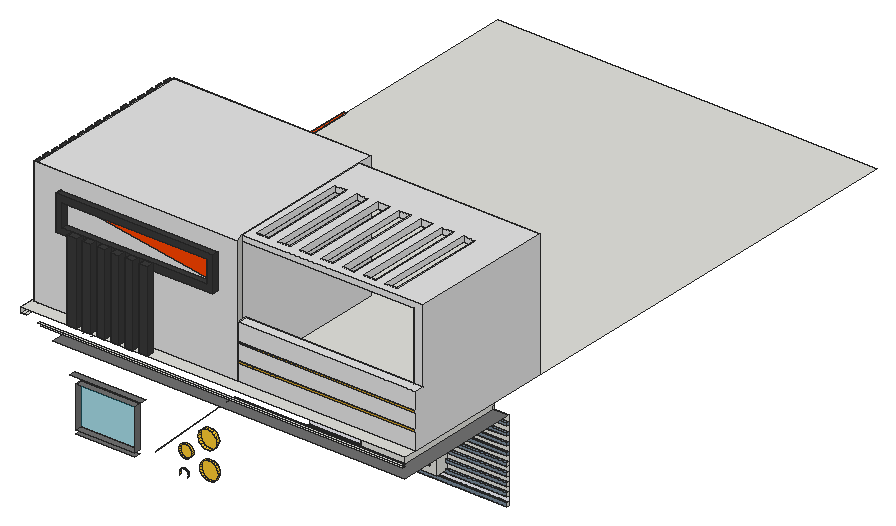
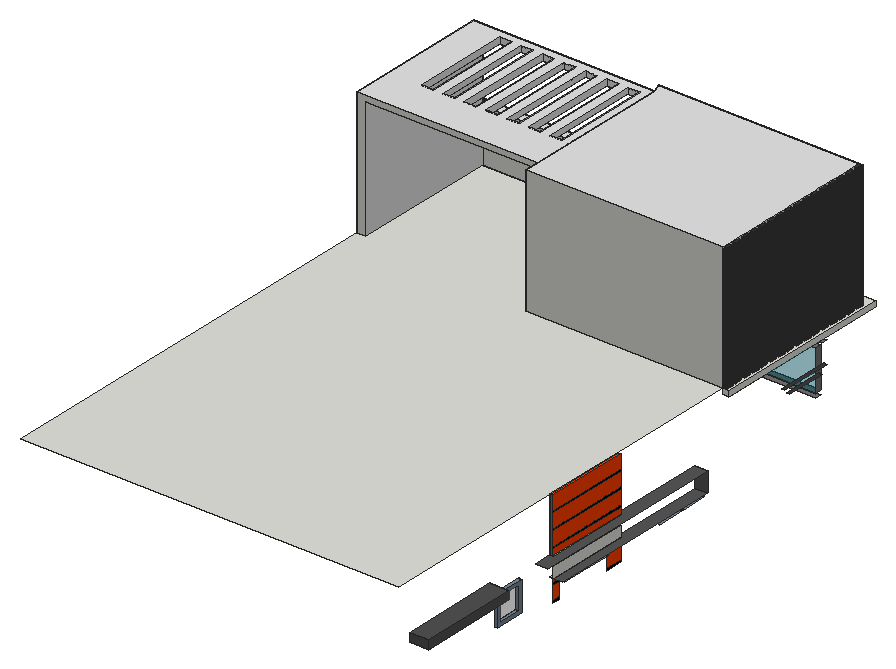
# SketchUp Ruby script. Lengths in inches.
U = 1.inch
M = Sketchup.active_model
def pt(a) = Geom::Point3d.new(a.map { |v| v * U })
def face(e, loops, mat)
  f = e.add_face(loops[0].map { |a| pt(a) })
  loops[1..].each { |l| e.add_face(l.map { |a| pt(a) }).erase! }
  f.material = f.back_material = mat if mat
  f
end
# faces: each face lists its corners as indices into pts; further lists are holes
def faces(e, pts, list, mat = nil) = list.each { |f| face(e, (f[0].is_a?(Array) ? f : [f]).map { |l| l.map { |i| pts[i] } }, mat) }
# xy, xz, yz: faces in a plane at the given z, y or x. An outline is a flat list of corners, or four numbers for a rectangle; further outlines are holes
def ring(l) = l.size == 4 ? [[l[0], l[1]], [l[2], l[1]], [l[2], l[3]], [l[0], l[3]]] : l.each_slice(2).to_a
def flat(e, list, mat, &to3) = list.each { |f| face(e, (f[0].is_a?(Array) ? f : [f]).map { |l| ring(l).map { |u, v| to3.(u, v) } }, mat) }
def xy(e, z, list, mat = nil) = flat(e, list, mat) { |x, y| [x, y, z] }
def xz(e, y, list, mat = nil) = flat(e, list, mat) { |x, z| [x, y, z] }
def yz(e, x, list, mat = nil) = flat(e, list, mat) { |y, z| [x, y, z] }
def lines(e, pts, list) = list.each { |a, b| e.add_line(pt(pts[a]), pt(pts[b])) }
# prism: a flat outline (further loops are holes) pulled along v
def prism(e, loops, v, mat = nil)
  f = face(e, loops, mat); d = Geom::Vector3d.new(v.map { |x| x * U })
  f.pushpull(f.normal.samedirection?(d) ? d.length : -d.length)
end
def box(e, o, s, mat = nil) = prism(e, [[o, [o[0] + s[0], o[1], o[2]], [o[0] + s[0], o[1] + s[1], o[2]], [o[0], o[1] + s[1], o[2]]]], [0, 0, s[2]], mat)
def at(x, y, z, deg = 0) = Geom::Transformation.translation(pt([x, y, z])) * Geom::Transformation.rotation(ORIGIN, Z_AXIS, deg.degrees)
def axes(o, x, y, z) = Geom::Transformation.new([*x, 0, *y, 0, *z, 0, *pt(o).to_a, 1])
def part(name) = M.definitions.add(name)
# library, detail: a bought-in or finely detailed component or shape, given as its bounding box
def library(name, o, s) = part(name).tap { |d| box(d.entities, o, s) }
def detail(e, o, s) = box(e.add_group.entities, o, s)
def put(e, d, t, mat = nil) = e.add_instance(d, t).tap { |i| i.material = mat if mat }
def group(e, t, mat = nil) = e.add_group.tap { |g| g.transformation = t; g.material = mat if mat }.entities
root = M.entities
M.materials.add("[0024_OrangeRed]").color = [255, 69, 0]
M.materials.add("[0045_Goldenrod]").color = [218, 165, 32]
M.materials.add("[0110_LightSlateGray]").color = [119, 136, 153]
M.materials.add("[0111_SlateGray]").color = [112, 128, 144]
M.materials.add("[0117_GhostWhite]").color = [248, 248, 255]
M.materials.add("[0135_DarkGray]").color = [81, 81, 81]
M.materials.add("[Color B05]").color = [255, 63, 0]
M.materials.add("[Color D04]").color = [255, 204, 50]
M.materials.add("[Color M05]").color = [114, 114, 114]
M.materials.add("[Color M06]").color = [86, 86, 86]
M.materials.add("[Color M07]").color = [58, 58, 58]
M.materials.add("[Color M09]").color = [0, 0, 0]
M.materials.add("[Polished Concrete Old]").color = [229, 229, 229]
M.materials.add("[Translucent Glass Gray]").color = [128, 128, 128]
M.materials["[Translucent Glass Gray]"].alpha = 0.5
M.materials.add("[Translucent Glass Tinted]").color = [4, 119, 142]
M.materials["[Translucent Glass Tinted]"].alpha = 0.48
xy(root,150.47,[[188.34,123.9375,363.6875,125.9375],[363.6875,123.9375,378,125.9375]],"[0110_LightSlateGray]")
xy(root,151.59,[[59.9,8,115.9,14]],"[Color M05]")
xy(root,153.53,[[188.34,123.9375,378,125.9375]],"[0110_LightSlateGray]")
xy(root,155.16,[[59.9,8,115.9,14]],"[Color M05]")
xy(root,159.03,[[188.34,123.9375,363.6875,125.9375],[363.6875,123.9375,378,125.9375]],"[0110_LightSlateGray]")
xy(root,160.2,[[246.52,113.9375,318.7,123.9375],[246.52,123.9375,318.7,125.9375]])
xy(root,161.99,[[15,420.33,18,448.89]],"[0110_LightSlateGray]")
xy(root,162.09,[[188.34,123.9375,246.52,125.9375],[318.7,123.9375,378,125.9375]],"[0110_LightSlateGray]")
xy(root,164.99,[[15,423.33,18,445.89]],"[0110_LightSlateGray]")
xy(root,165.42,[[15,203.12,18,226.79],[15,229.5,18,255.87]],"[0110_LightSlateGray]")
xy(root,166.2,[[252.52,113.9375,312.7,125.9375]])
xy(root,167.59,[[188.34,123.9375,246.52,125.9375],[318.7,123.9375,363.6875,125.9375],[363.6875,123.9375,378,125.9375]],"[0110_LightSlateGray]")
xy(root,168.375,[[12,321.75,15,345.13],[12,347.25,15,372.75]],"[0110_LightSlateGray]")
xy(root,168.42,[[15,200.12,18,258.87]],"[0110_LightSlateGray]")
xy(root,170.66,[[188.34,123.9375,246.52,125.9375],[318.7,123.9375,378,125.9375]],"[0110_LightSlateGray]")
xy(root,171.375,[[12,318.75,15,375.75]],"[0110_LightSlateGray]")
xy(root,174.92,[[15,302.36,18,382.63]])
xy(root,174.92,[[6,209.95,6,382.63,15,382.63,15,302.36,18,302.36,18,209.95]],"[Color M06]")
xy(root,176.15,[[188.34,123.9375,246.52,125.9375],[318.7,123.9375,363.6875,125.9375],[363.6875,123.9375,378,125.9375]],"[0110_LightSlateGray]")
xy(root,179.22,[[188.34,123.9375,246.52,125.9375]])
xy(root,179.22,[[318.7,123.9375,378,125.9375]],"[0110_LightSlateGray]")
xy(root,184.72,[[188.34,123.9375,246.52,125.9375],[318.7,123.9375,363.6875,125.9375],[363.6875,123.9375,378,125.9375]],"[0110_LightSlateGray]")
xy(root,187.55,[[15,423.33,18,445.89]])
xy(root,187.78,[[188.34,123.9375,246.52,125.9375]])
xy(root,187.78,[[318.7,123.9375,378,125.9375]],"[0110_LightSlateGray]")
xy(root,190.1,[[15,466.73,18,500.63],[15,503.73,18,540.73]],"[0135_DarkGray]")
xy(root,190.55,[[15,420.33,18,448.89]],"[0110_LightSlateGray]")
xy(root,193.1,[[0,453.79,0,549.98,18,549.98,18,543.73,15,543.73,15,463.73,18,463.73,18,453.79]],"[0135_DarkGray]")
xy(root,193.28,[[188.34,123.9375,246.52,125.9375],[318.7,123.9375,363.6875,125.9375],[363.6875,123.9375,378,125.9375]],"[0110_LightSlateGray]")
xy(root,194.12,[[59.9,8,115.9,14]],"[Color M05]")
xy(root,194.23,[[15,302.36,18,382.63]])
xy(root,194.23,[[6,209.95,18,209.95,18,302.36,15,302.36,15,382.63,18,382.63,18,399.82,6,399.82]],"[Color M06]")
xy(root,196.34,[[188.34,123.9375,246.52,125.9375]])
xy(root,196.34,[[318.7,123.9375,378,125.9375]],"[0110_LightSlateGray]")
xy(root,200.12,[[53.9,8,121.9,14]],"[Color M05]")
xy(root,201.17,[[0,453.79,18,549.98]],"[0135_DarkGray]")
xy(root,201.84,[[318.7,123.9375,363.6875,125.9375],[363.6875,123.9375,378,125.9375]],"[0110_LightSlateGray]")
xy(root,201.84,[[188.34,123.9375,246.52,125.9375]],"[0111_SlateGray]")
xy(root,203.27,[[252.52,113.9375,312.7,125.9375]])
xy(root,204.91,[[318.7,123.9375,378,125.9375]],"[0110_LightSlateGray]")
xy(root,204.91,[[188.34,123.9375,246.52,125.9375]],"[0111_SlateGray]")
xy(root,209.27,[[246.52,113.9375,318.7,125.9375]])
xy(root,210.4,[[188.34,123.9375,363.6875,125.9375],[363.6875,123.9375,378,125.9375]],"[0110_LightSlateGray]")
xy(root,211.37,[[12,66.99,15,104.86]],"[Color M07]")
xy(root,213.47,[[188.34,123.9375,378,125.9375]],"[0110_LightSlateGray]")
xy(root,217.37,[[12,60.99,15,110.86]],"[Color M07]")
xy(root,218.97,[[188.34,123.9375,363.6875,125.9375],[363.6875,123.9375,378,125.9375]],"[0110_LightSlateGray]")
xy(root,222.03,[[188.34,123.9375,378,125.9375]],"[0110_LightSlateGray]")
xy(root,227.53,[[188.34,123.9375,363.6875,125.9375]],"[0110_LightSlateGray]")
xy(root,227.53,[[42.91,2,42.91,14,201.375,14,201.375,20,363.6875,20,363.6875,125.9375,378,125.9375,378,2]],"[Color M05]")
xy(root,230.84,[[188.34,123.9375,363.6875,125.9375]])
xy(root,236.34,[[188.34,123.9375,363.6875,125.9375]],"[0110_LightSlateGray]")
xy(root,238.03,[[32.7,0,378,2]])
xy(root,239.39,[[30.46,0,378,2]])
xy(root,240,[[27,20,27,125.9375,188.34,125.9375,188.34,123.9375,363.6875,123.9375,363.6875,20]],"[Polished Concrete Old]")
xy(root,240.8125,[[12,2,15,175.3125],[15,2,18,175.3125],[12,175.3125,18,177.0625]])
xy(root,246,[[[12,2,378,2,378,14.84,15,14.84,15,21.19,18,21.19,18,25.15,15,25.15,15,31.5,18,31.5,18,35.46,15,35.46,15,41.81,18,41.81,18,45.78,15,45.78,15,52.13,18,52.13,18,56.09,15,56.09,15,62.44,18,62.44,18,66.4,15,66.4,15,72.75,18,72.75,18,76.71,15,76.71,15,83.06,18,83.06,18,87.03,15,87.03,15,93.38,18,93.38,18,97.34,15,97.34,15,103.69,18,103.69,18,107.65,15,107.65,15,114,18,114,18,117.96,15,117.96,15,124.31,18,124.31,18,128.28,15,128.28,15,134.63,18,134.63,18,138.59,15,138.59,15,144.94,18,144.94,18,148.9,15,148.9,15,155.25,18,155.25,18,159.21,15,159.21,15,165.56,18,165.56,18,169.53,15,169.53,15,175.88,18,175.88,18,176.98,205.83,176.98,205.83,23.84,209.18,23.84,209.18,24.34,369,24.34,369,162.88,378,162.88,378,563,18,563,18,177.0625,12,177.0625],[56.4375,2.09,66.15,8.84],[84.32,2.09,92.33,8.84],[97.82,2.09,105.83,8.84],[111.32,2.09,119.33,8.84],[124.82,2.09,132.83,8.84],[70.82,2.09,78.83,8.84]],[15,14.84,18,21.19],[18,14.84,27,23.84],[27,14.84,209.18,14.84,205.83,23.84,27,23.84],[209.18,14.84,209.18,23.84,205.83,23.84],
  [209.18,14.84,377.18,24.34],[377.18,14.84,378,24.34],[18,23.84,27,176.98],[27,23.84,205.83,176.98],[369,24.34,378,162.88],
  [15,25.15,18,31.5],[15,35.46,18,41.81],[15,45.78,18,52.13],[15,56.09,18,62.44],[15,66.4,18,72.75],
  [15,76.71,18,83.06],[15,87.03,18,93.38],[15,97.34,18,103.69],[15,107.65,18,114],[15,117.96,18,124.31],
  [15,128.28,18,134.63],[15,138.59,18,144.94],[15,148.9,18,155.25],[15,159.21,18,165.56],[15,169.53,18,175.88]])
xy(root,246,[[15,302.36,18,382.63]],"[0024_OrangeRed]")
xy(root,262.33,[[209.18,13.84,378,14.84]])
xy(root,264.09,[[209.18,13.84,378,14.84]])
xy(root,278.67,[[209.18,13.84,378,14.84]])
xy(root,280.32,[[209.18,13.84,378,14.84]])
xy(root,296.375,[[209.18,14.84,378,14.84,378,23.84,369.17,23.84,369,24.34,209.18,24.34]],"[Polished Concrete Old]")
xy(root,316.27,[[40.375,8.84,189.625,14.84]],"[Color M07]")
xy(root,322.27,[[56.4375,2.09,66.15,8.84],[70.82,2.09,78.83,8.84],[84.32,2.09,92.33,8.84],[97.82,2.09,105.83,8.84],[111.32,2.09,119.33,8.84],
  [124.82,2.09,132.83,8.84],[46.375,8.84,183.625,14.84]],"[Color M07]")
xy(root,343.64,[[46.375,8.84,183.625,14.84]],"[Color M07]")
xy(root,349.64,[[40.375,8.84,189.625,14.84]],"[Color M07]")
xy(root,360.43,[[179.6875,24.34,205.83,162.88]])
xy(root,360.43,[[[205.83,23.84,205.83,162.88,369,162.88,369,24.34,369.17,23.84],[213.22,31.79,224.41,124.92],[233.6,31.79,244.79,124.92],[253.97,31.79,265.16,124.92],[274.35,31.79,285.54,124.92],[294.72,31.79,305.91,124.92],[315.1,31.79,326.29,124.92],[335.47,31.79,346.66,124.92]]],"[Polished Concrete Old]")
xy(root,366,[[15,14.84,18,21.19],[15,25.15,18,31.5],[15,35.46,18,41.81],[15,45.78,18,52.13],[15,56.09,18,62.44],
  [15,66.4,18,72.75],[15,76.71,18,83.06],[15,87.03,18,93.38],[15,97.34,18,103.69],[15,107.65,18,114],
  [15,117.96,18,124.31],[15,128.28,18,134.63],[15,138.59,18,144.94],[15,148.9,18,155.25],[15,159.21,18,165.56],
  [15,169.53,18,175.88]],"[Color M07]")
xy(root,366,[[18,14.84,209.18,14.84,205.83,23.84,205.83,176.98,18,176.98],[[205.83,23.84,378,162.88],[335.47,31.79,346.66,124.92],[213.22,31.79,224.41,124.92],[233.6,31.79,244.79,124.92],[253.97,31.79,265.16,124.92],[274.35,31.79,285.54,124.92],[294.72,31.79,305.91,124.92],[315.1,31.79,326.29,124.92]]],"[Polished Concrete Old]")
xz(root,2.09,[[56.4375,246,66.15,322.27],[70.82,246,78.83,322.27],[84.32,246,92.33,322.27],[97.82,246,105.83,322.27],[111.32,246,119.33,322.27],
  [124.82,246,132.83,322.27]],"[Color M07]")
xz(root,8.84,[[56.4375,246,66.15,316.27],[70.82,246,78.83,316.27],[84.32,246,92.33,316.27],[97.82,246,105.83,316.27],[111.32,246,119.33,316.27],
  [124.82,246,132.83,316.27],[56.4375,316.27,66.15,322.27],[70.82,316.27,78.83,322.27],[84.32,316.27,92.33,322.27],[97.82,316.27,105.83,322.27],
  [111.32,316.27,119.33,322.27],[124.82,316.27,132.83,322.27]])
xz(root,8.84,[[40.375,316.27,56.4375,316.27,56.4375,322.27,46.375,322.27,46.375,343.64,183.625,343.64,183.625,322.27,132.83,322.27,132.83,316.27,189.625,316.27,189.625,349.64,40.375,349.64],[66.15,316.27,70.82,322.27],[78.83,316.27,84.32,322.27],[92.33,316.27,97.82,322.27],[105.83,316.27,111.32,322.27],
  [119.33,316.27,124.82,322.27]],"[Color M07]")
xz(root,12.875,[[161.99,165.1,163.61,165.31,165.11,165.93,166.41,166.93,167.4,168.22,168.03,169.73,168.24,171.35,168.03,172.96,167.4,174.47,166.41,175.77,165.11,176.76,163.61,177.38,161.99,177.6,160.37,177.38,158.86,176.76,157.57,175.77,156.58,174.47,155.95,172.96,155.74,171.35,155.95,169.73,156.58,168.22,157.57,166.93,158.86,165.93,160.37,165.31]],"[Color D04]")
xz(root,13.125,[[184.53,153.64,186.82,153.94,188.95,154.83,190.79,156.24,192.19,158.07,193.08,160.2,193.38,162.49,193.08,164.79,192.19,166.92,190.79,168.75,188.95,170.16,186.82,171.05,184.53,171.35,182.23,171.05,180.1,170.16,178.27,168.75,176.86,166.92,175.97,164.79,175.67,162.49,175.97,160.2,176.86,158.07,178.27,156.24,180.1,154.83,182.23,153.94]],"[Color D04]")
xz(root,13.84,[[209.18,262.33,378,264.09],[209.18,278.67,378,280.32]],"[0045_Goldenrod]")
xz(root,14,[[59.9,155.16,115.9,194.12]],"[Translucent Glass Tinted]")
xz(root,14.25,[[182.83,179.81,185.13,180.11,187.27,181,189.11,182.41,190.52,184.25,191.41,186.39,191.71,188.68,191.41,190.98,190.52,193.12,189.11,194.96,187.27,196.37,185.13,197.26,182.83,197.56,180.54,197.26,178.4,196.37,176.56,194.96,175.15,193.12,174.26,190.98,173.96,188.68,174.26,186.39,175.15,184.25,176.56,182.41,178.4,181,180.54,180.11]],"[Color D04]")
xz(root,14.84,[[183.625,322.27,183.625,343.64,46.375,343.64]],"[0024_OrangeRed]")
xz(root,14.84,[[[15,246,209.18,366],[40.375,316.27,189.625,349.64]],[209.18,246,378,262.33],[209.18,264.09,378,278.67],[209.18,280.32,378,296.375],[46.375,322.27,183.625,322.27,46.375,343.64]],"[Polished Concrete Old]")
xz(root,21.19,[[15,246,18,366]],"[Color M07]")
xz(root,23.84,[[369.17,296.375,378,296.375,378,366,205.83,366,205.83,360.43,369.17,360.43]],"[Polished Concrete Old]")
xz(root,24.34,[[209.18,246,369,296.375],[369,246,377.18,296.375]])
xz(root,25.15,[[15,246,18,366]],"[Color M07]")
xz(root,31.5,[[15,246,18,366]],"[Color M07]")
xz(root,31.79,[[213.22,360.43,224.41,366],[233.6,360.43,244.79,366],[253.97,360.43,265.16,366],[274.35,360.43,285.54,366],[294.72,360.43,305.91,366],
  [315.1,360.43,326.29,366],[335.47,360.43,346.66,366]],"[Polished Concrete Old]")
xz(root,35.46,[[15,246,18,366]],"[Color M07]")
xz(root,41.81,[[15,246,18,366]],"[Color M07]")
xz(root,45.78,[[15,246,18,366]],"[Color M07]")
xz(root,52.13,[[15,246,18,366]],"[Color M07]")
xz(root,56.09,[[15,246,18,366]],"[Color M07]")
xz(root,62.44,[[15,246,18,366]],"[Color M07]")
xz(root,66.4,[[15,246,18,366]],"[Color M07]")
xz(root,72.75,[[15,246,18,366]],"[Color M07]")
xz(root,76.71,[[15,246,18,366]],"[Color M07]")
xz(root,83.06,[[15,246,18,366]],"[Color M07]")
xz(root,87.03,[[15,246,18,366]],"[Color M07]")
xz(root,93.38,[[15,246,18,366]],"[Color M07]")
xz(root,97.34,[[15,246,18,366]],"[Color M07]")
xz(root,103.69,[[15,246,18,366]],"[Color M07]")
xz(root,107.65,[[15,246,18,366]],"[Color M07]")
xz(root,113.9375,[[[246.52,160.2,318.7,209.27],[252.52,166.2,312.7,203.27]]])
xz(root,114,[[15,246,18,366]],"[Color M07]")
xz(root,117.96,[[15,246,18,366]],"[Color M07]")
xz(root,123.9375,[[188.34,150.47,378,153.53],[188.34,159.03,378,159.03,378,162.09,318.7,162.09,318.7,160.2,246.52,160.2,246.52,162.09,188.34,162.09],[188.34,167.59,246.52,170.66],[318.7,167.59,378,170.66],[188.34,176.15,246.52,179.22],
  [318.7,176.15,378,179.22],[188.34,184.72,246.52,187.78],[318.7,184.72,378,187.78],[188.34,193.28,246.52,196.34],[318.7,193.28,378,196.34],
  [318.7,201.84,378,204.91],[188.34,210.4,378,213.47],[188.34,218.97,378,222.03],[188.34,227.53,363.6875,230.84],[188.34,236.34,363.6875,240]],"[0110_LightSlateGray]")
xz(root,123.9375,[[188.34,201.84,246.52,204.91]],"[0111_SlateGray]")
xz(root,124.31,[[15,246,18,366]],"[Color M07]")
xz(root,124.92,[[213.22,360.43,224.41,366],[233.6,360.43,244.79,366],[253.97,360.43,265.16,366],[274.35,360.43,285.54,366],[294.72,360.43,305.91,366],
  [315.1,360.43,326.29,366],[335.47,360.43,346.66,366]],"[Polished Concrete Old]")
xz(root,125.9375,[[188.34,150.47,378,153.53],[188.34,159.03,188.34,162.09,246.52,162.09,246.52,160.2,318.7,160.2,318.7,162.09,378,162.09,378,159.03],[188.34,162.09,246.52,167.59],[246.52,162.09,318.7,162.09,318.7,167.59,312.7,167.59,312.7,166.2,252.52,166.2,252.52,167.59,246.52,167.59],[318.7,162.09,378,167.59],
  [252.52,166.2,312.7,203.27],[188.34,167.59,246.52,170.66],[318.7,167.59,378,170.66],[188.34,170.66,246.52,176.15],[246.52,170.66,252.52,176.15],
  [312.7,170.66,318.7,176.15],[318.7,170.66,378,176.15],[188.34,176.15,246.52,179.22],[318.7,176.15,378,179.22],[188.34,179.22,246.52,184.72],
  [246.52,179.22,252.52,184.72],[312.7,179.22,318.7,184.72],[318.7,179.22,378,184.72],[188.34,184.72,246.52,187.78],[318.7,184.72,378,187.78],
  [188.34,187.78,246.52,193.28],[246.52,187.78,252.52,193.28],[312.7,187.78,318.7,193.28],[318.7,187.78,378,193.28],[188.34,193.28,246.52,196.34],
  [318.7,193.28,378,196.34],[246.52,196.34,252.52,201.84],[312.7,196.34,318.7,201.84],[318.7,196.34,378,201.84],[318.7,201.84,378,204.91],
  [188.34,204.91,246.52,204.91,246.52,209.27,318.7,209.27,318.7,204.91,378,204.91,378,210.4,188.34,210.4],[246.52,204.91,318.7,209.27],[188.34,210.4,378,213.47],[188.34,213.47,378,218.97],[188.34,218.97,378,222.03],
  [188.34,222.03,378,227.53],[188.34,227.53,363.6875,230.84],[188.34,230.84,363.6875,236.34]])
xz(root,125.9375,[[188.34,153.53,378,159.03],[188.34,196.34,246.52,201.84]],"[0117_GhostWhite]")
xz(root,128.28,[[15,246,18,366]],"[Color M07]")
xz(root,134.63,[[15,246,18,366]],"[Color M07]")
xz(root,138.59,[[15,246,18,366]],"[Color M07]")
xz(root,144.94,[[15,246,18,366]],"[Color M07]")
xz(root,148.9,[[15,246,18,366]],"[Color M07]")
xz(root,155.25,[[15,246,18,366]],"[Color M07]")
xz(root,159.21,[[15,246,18,366]],"[Color M07]")
xz(root,162.88,[[369,246,369,360.43,205.83,360.43,205.83,366,378,366,378,246]])
xz(root,165.56,[[15,246,18,366]],"[Color M07]")
xz(root,169.53,[[15,246,18,366]],"[Color M07]")
xz(root,175.88,[[15,246,18,366]],"[Color M07]")
xz(root,176.98,[[18,246,205.83,366]])
xz(root,177.0625,[[12,240.8125,18,246]])
xz(root,209.95,[[6,174.92,18,194.23]],"[Color M06]")
xz(root,302.36,[[15,194.23,18,246]],"[0024_OrangeRed]")
xz(root,382.63,[[15,194.23,18,246]],"[0024_OrangeRed]")
xz(root,420.33,[[15,161.99,18,190.55]],"[0110_LightSlateGray]")
xz(root,423.33,[[15,164.99,18,187.55]],"[0110_LightSlateGray]")
xz(root,445.89,[[15,164.99,18,187.55]],"[0110_LightSlateGray]")
xz(root,448.89,[[15,161.99,18,190.55]],"[0110_LightSlateGray]")
xz(root,453.79,[[0,193.1,18,201.17]],"[0135_DarkGray]")
xz(root,549.98,[[0,193.1,18,201.17]],"[0135_DarkGray]")
yz(root,0,[[453.79,193.1,549.98,201.17]],"[0135_DarkGray]")
yz(root,12,[[2,240.8125,177.0625,246]])
yz(root,15,[[302.36,174.92,382.63,184.5],[302.36,186.75,382.63,194.23]])
yz(root,15,[[375.75,156,382.63,169.125]],"[0024_OrangeRed]")
yz(root,15,[[[420.33,161.99,448.89,190.55],[423.33,164.99,445.89,187.55]]],"[0110_LightSlateGray]")
yz(root,15,[[302.36,156,318.75,169.125],[302.36,171.375,382.63,174.92],[302.36,194.23,382.63,199.875],[302.36,202.125,382.63,215.25],[302.36,217.5,382.63,230.625],
  [302.36,232.875,382.63,246]],"[Color B05]")
yz(root,15,[[14.84,246,21.19,366],[25.15,246,31.5,366],[35.46,246,41.81,366],[45.78,246,52.13,366],[56.09,246,62.44,366],
  [66.4,246,72.75,366],[76.71,246,83.06,366],[87.03,246,93.38,366],[97.34,246,103.69,366],[107.65,246,114,366],
  [117.96,246,124.31,366],[128.28,246,134.63,366],[138.59,246,144.94,366],[148.9,246,155.25,366],[159.21,246,165.56,366],
  [169.53,246,175.88,366]],"[Color M07]")
yz(root,15,[[302.36,153.75,318.75,156],[375.75,153.75,382.63,156],[302.36,169.125,318.75,171.375],[375.75,169.125,382.63,171.375],[302.36,199.875,382.63,202.125],
  [302.36,215.25,382.63,217.5],[302.36,230.625,382.63,232.875]],"[Color M09]")
yz(root,18,[[302.36,194.23,382.63,246],[21.19,246,25.15,366],[25.15,246,31.5,366],[31.5,246,35.46,366],[35.46,246,41.81,366],
  [41.81,246,45.78,366],[45.78,246,52.13,366],[52.13,246,56.09,366],[56.09,246,62.44,366],[62.44,246,66.4,366],
  [66.4,246,72.75,366],[72.75,246,76.71,366],[76.71,246,83.06,366],[83.06,246,87.03,366],[87.03,246,93.38,366],
  [93.38,246,97.34,366],[97.34,246,103.69,366],[103.69,246,107.65,366],[107.65,246,114,366],[114,246,117.96,366],
  [117.96,246,124.31,366],[124.31,246,128.28,366],[128.28,246,134.63,366],[134.63,246,138.59,366],[138.59,246,144.94,366],
  [144.94,246,148.9,366],[148.9,246,155.25,366],[155.25,246,159.21,366],[159.21,246,165.56,366],[165.56,246,169.53,366],
  [169.53,246,175.88,366],[175.88,246,176.98,366]])
yz(root,18,[[423.33,164.99,445.89,187.55]],"[Translucent Glass Gray]")
yz(root,40.375,[[8.84,316.27,14.84,349.64]],"[Color M07]")
yz(root,46.375,[[8.84,322.27,14.84,343.64]],"[Color M07]")
yz(root,56.4375,[[2.09,246,8.84,322.27]],"[Color M07]")
yz(root,59.9,[[8,155.16,14,194.12]],"[Color M05]")
yz(root,66.15,[[2.09,246,8.84,322.27]],"[Color M07]")
yz(root,70.82,[[2.09,246,8.84,322.27]],"[Color M07]")
yz(root,78.83,[[2.09,246,8.84,322.27]],"[Color M07]")
yz(root,84.32,[[2.09,246,8.84,322.27]],"[Color M07]")
yz(root,92.33,[[2.09,246,8.84,322.27]],"[Color M07]")
yz(root,97.82,[[2.09,246,8.84,322.27]],"[Color M07]")
yz(root,105.83,[[2.09,246,8.84,322.27]],"[Color M07]")
yz(root,111.32,[[2.09,246,8.84,322.27]],"[Color M07]")
yz(root,115.9,[[8,155.16,14,194.12]],"[Color M05]")
yz(root,119.33,[[2.09,246,8.84,322.27]],"[Color M07]")
yz(root,124.82,[[2.09,246,8.84,322.27]],"[Color M07]")
yz(root,132.83,[[2.09,246,8.84,322.27]],"[Color M07]")
yz(root,183.625,[[8.84,322.27,14.84,343.64]],"[Color M07]")
yz(root,188.34,[[123.9375,150.47,125.9375,153.53],[123.9375,159.03,125.9375,162.09],[123.9375,167.59,125.9375,170.66],[123.9375,176.15,125.9375,179.22],[123.9375,184.72,125.9375,187.78],
  [123.9375,193.28,125.9375,196.34],[123.9375,210.4,125.9375,213.47],[123.9375,218.97,125.9375,222.03],[123.9375,227.53,125.9375,230.84],[123.9375,236.34,125.9375,240]],"[0110_LightSlateGray]")
yz(root,188.34,[[123.9375,201.84,125.9375,204.91]],"[0111_SlateGray]")
yz(root,189.625,[[8.84,316.27,14.84,349.64]],"[Color M07]")
yz(root,205.83,[[23.84,360.43,162.88,366]])
yz(root,205.83,[[23.84,246,176.98,246,176.98,366,162.88,366,162.88,360.43,23.84,360.43]],"[Polished Concrete Old]")
yz(root,209.18,[[14.84,246,24.34,296.375],[13.84,262.33,14.84,264.09],[13.84,278.67,14.84,280.32]])
yz(root,213.22,[[31.79,360.43,124.92,366]],"[Polished Concrete Old]")
yz(root,224.41,[[31.79,360.43,124.92,366]],"[Polished Concrete Old]")
yz(root,233.6,[[31.79,360.43,124.92,366]],"[Polished Concrete Old]")
yz(root,244.79,[[31.79,360.43,124.92,366]],"[Polished Concrete Old]")
yz(root,246.52,[[113.9375,160.2,113.9375,209.27,125.9375,209.27,125.9375,204.91,123.9375,204.91,123.9375,201.84,125.9375,201.84,125.9375,196.34,123.9375,196.34,123.9375,193.28,125.9375,193.28,125.9375,187.78,123.9375,187.78,123.9375,184.72,125.9375,184.72,125.9375,179.22,123.9375,179.22,123.9375,176.15,125.9375,176.15,125.9375,170.66,123.9375,170.66,123.9375,167.59,125.9375,167.59,125.9375,162.09,123.9375,162.09,123.9375,160.2],[123.9375,160.2,125.9375,162.09],[123.9375,167.59,125.9375,170.66],[123.9375,176.15,125.9375,179.22],[123.9375,184.72,125.9375,187.78],
  [123.9375,193.28,125.9375,196.34]])
yz(root,252.52,[[113.9375,166.2,125.9375,203.27]])
yz(root,253.97,[[31.79,360.43,124.92,366]],"[Polished Concrete Old]")
yz(root,265.16,[[31.79,360.43,124.92,366]],"[Polished Concrete Old]")
yz(root,274.35,[[31.79,360.43,124.92,366]],"[Polished Concrete Old]")
yz(root,285.54,[[31.79,360.43,124.92,366]],"[Polished Concrete Old]")
yz(root,294.72,[[31.79,360.43,124.92,366]],"[Polished Concrete Old]")
yz(root,305.91,[[31.79,360.43,124.92,366]],"[Polished Concrete Old]")
yz(root,312.7,[[113.9375,166.2,125.9375,203.27]])
yz(root,315.1,[[31.79,360.43,124.92,366]],"[Polished Concrete Old]")
yz(root,318.7,[[113.9375,160.2,123.9375,160.2,123.9375,162.09,125.9375,162.09,125.9375,167.59,123.9375,167.59,123.9375,170.66,125.9375,170.66,125.9375,176.15,123.9375,176.15,123.9375,179.22,125.9375,179.22,125.9375,184.72,123.9375,184.72,123.9375,187.78,125.9375,187.78,125.9375,193.28,123.9375,193.28,123.9375,196.34,125.9375,196.34,125.9375,201.84,123.9375,201.84,123.9375,204.91,125.9375,204.91,125.9375,209.27,113.9375,209.27],[123.9375,160.2,125.9375,162.09],[123.9375,167.59,125.9375,170.66],[123.9375,176.15,125.9375,179.22],[123.9375,184.72,125.9375,187.78],
  [123.9375,193.28,125.9375,196.34],[123.9375,201.84,125.9375,204.91]])
yz(root,326.29,[[31.79,360.43,124.92,366]],"[Polished Concrete Old]")
yz(root,335.47,[[31.79,360.43,124.92,366]],"[Polished Concrete Old]")
yz(root,346.66,[[31.79,360.43,124.92,366]],"[Polished Concrete Old]")
yz(root,363.6875,[[20,227.53,20,240,123.9375,240,123.9375,236.34,125.9375,236.34,125.9375,230.84,123.9375,230.84,123.9375,227.53],[123.9375,227.53,125.9375,230.84]])
yz(root,369,[[24.34,246,162.88,360.43]],"[Polished Concrete Old]")
yz(root,378,[[123.9375,150.47,125.9375,153.53],[123.9375,159.03,125.9375,162.09],[123.9375,167.59,125.9375,170.66],[123.9375,176.15,125.9375,179.22],[123.9375,184.72,125.9375,187.78]])
yz(root,378,[[123.9375,193.28,125.9375,196.34],[123.9375,201.84,125.9375,204.91],[123.9375,210.4,125.9375,213.47],[123.9375,218.97,125.9375,222.03]],"[0110_LightSlateGray]")
yz(root,378,[[14.84,246,162.88,246,162.88,366,23.84,366,23.84,296.375,14.84,296.375,14.84,280.32,13.84,280.32,13.84,278.67,14.84,278.67,14.84,264.09,13.84,264.09,13.84,262.33,14.84,262.33]],"[Polished Concrete Old]")
p = [[156.58,11,150.79],[156.99,11,149.78],[156.99,12.0625,149.78],[156.58,12.0625,150.79],[164.25,11,149.78],[164.67,11,150.79],
  [164.67,12.0625,150.79],[164.25,12.0625,149.78],[156.43,11,151.87],[156.43,12.0625,151.87],[164.81,11,151.87],[164.81,12.0625,151.87],
  [156.58,11,152.95],[156.58,12.0625,152.95],[164.67,11,152.95],[164.67,12.0625,152.95],[156.99,11,153.96],[156.99,12.0625,153.96],
  [164.25,11,153.96],[164.25,12.0625,153.96],[182.23,11,153.94],[184.53,11,153.64],[184.53,13.125,153.64],[182.23,13.125,153.94],
  [186.82,11,153.94],[186.82,13.125,153.94],[180.1,11,154.83],[180.1,13.125,154.83],[188.95,11,154.83],[188.95,13.125,154.83],
  [157.66,11,154.83],[157.66,12.0625,154.83],[163.58,11,154.83],[163.58,12.0625,154.83],[158.53,11,155.5],[158.53,12.0625,155.5],
  [162.71,11,155.5],[162.71,12.0625,155.5],[178.27,11,156.24],[178.27,13.125,156.24],[190.79,11,156.24],[190.79,13.125,156.24],
  [159.54,11,155.92],[159.54,12.0625,155.92],[161.7,11,155.92],[161.7,12.0625,155.92],[160.62,11,156.06],[160.62,12.0625,156.06],
  [176.86,11,158.07],[176.86,13.125,158.07],[192.19,11,158.07],[192.19,13.125,158.07],[175.97,11,160.2],[175.97,13.125,160.2],
  [193.08,11,160.2],[193.08,13.125,160.2],[175.67,11,162.49],[175.67,13.125,162.49],[193.38,11,162.49],[193.38,13.125,162.49],
  [201.375,14,227.53],[133.54,14,160.93],[133.54,11,160.93],[201.375,11,227.53],[175.97,11,164.79],[175.97,13.125,164.79],
  [193.08,11,164.79],[193.08,13.125,164.79],[176.86,11,166.92],[176.86,13.125,166.92],[192.19,11,166.92],[192.19,13.125,166.92],
  [160.37,11,165.31],[161.99,11,165.1],[161.99,12.875,165.1],[160.37,12.875,165.31],[163.61,11,165.31],[163.61,12.875,165.31],
  [158.86,11,165.93],[158.86,12.875,165.93],[165.11,11,165.93],[165.11,12.875,165.93],[157.57,11,166.93],[157.57,12.875,166.93],
  [166.41,11,166.93],[166.41,12.875,166.93],[156.58,11,168.22],[156.58,12.875,168.22],[167.4,11,168.22],[167.4,12.875,168.22],
  [178.27,11,168.75],[178.27,13.125,168.75],[190.79,11,168.75],[190.79,13.125,168.75],[155.95,11,169.73],[155.95,12.875,169.73],
  [168.03,11,169.73],[168.03,12.875,169.73],[180.1,11,170.16],[180.1,13.125,170.16],[188.95,11,170.16],[188.95,13.125,170.16],
  [155.74,11,171.35],[155.74,12.875,171.35],[168.24,11,171.35],[168.24,12.875,171.35],[182.23,11,171.05],[182.23,13.125,171.05],
  [186.82,11,171.05],[186.82,13.125,171.05],[184.53,11,171.35],[184.53,13.125,171.35],[155.95,11,172.96],[155.95,12.875,172.96],
  [168.03,11,172.96],[168.03,12.875,172.96],[156.58,11,174.47],[156.58,12.875,174.47],[167.4,11,174.47],[167.4,12.875,174.47],
  [157.57,11,175.77],[157.57,12.875,175.77],[166.41,11,175.77],[166.41,12.875,175.77],[158.86,11,176.76],[158.86,12.875,176.76],
  [165.11,11,176.76],[165.11,12.875,176.76],[160.37,11,177.38],[160.37,12.875,177.38],[163.61,11,177.38],[163.61,12.875,177.38],
  [161.99,11,177.6],[161.99,12.875,177.6],[180.54,11,180.11],[182.83,11,179.81],[182.83,14.25,179.81],[180.54,14.25,180.11],
  [185.13,11,180.11],[185.13,14.25,180.11],[178.4,11,181],[178.4,14.25,181],[187.27,11,181],[187.27,14.25,181],
  [176.56,11,182.41],[176.56,14.25,182.41],[189.11,11,182.41],[189.11,14.25,182.41],[175.15,11,184.25],[175.15,14.25,184.25],
  [190.52,11,184.25],[190.52,14.25,184.25],[174.26,11,186.39],[174.26,14.25,186.39],[191.41,11,186.39],[191.41,14.25,186.39],
  [173.96,11,188.68],[173.96,14.25,188.68],[191.71,11,188.68],[191.71,14.25,188.68],[174.26,11,190.98],[174.26,14.25,190.98],
  [191.41,11,190.98],[191.41,14.25,190.98],[175.15,11,193.12],[175.15,14.25,193.12],[190.52,11,193.12],[190.52,14.25,193.12],
  [176.56,11,194.96],[176.56,14.25,194.96],[189.11,11,194.96],[189.11,14.25,194.96],[178.4,11,196.37],[178.4,14.25,196.37],
  [187.27,11,196.37],[187.27,14.25,196.37],[180.54,11,197.26],[180.54,14.25,197.26],[185.13,11,197.26],[185.13,14.25,197.26],
  [182.83,11,197.56],[182.83,14.25,197.56],[209.18,14.84,246],[205.83,23.84,246],[205.83,23.84,360.43],[205.83,23.84,366],
  [209.18,14.84,366],[209.18,14.84,296.375],[209.18,14.84,280.32],[209.18,14.84,278.67],[209.18,14.84,264.09],[209.18,14.84,262.33],
  [369.17,23.84,360.43],[369,24.34,360.43],[369,24.34,296.375],[369.17,23.84,296.375],[27,125.9375,240],[27,134.9375,240],
  [27,371,240],[27,380,240],[369,162.71,360.43],[369,162.71,366],[377.18,162.71,360.43],[378,162.71,360.43],
  [369,162.88,366],[378,23.84,296.375],[378,24.34,296.375],[70.82,8.84,243.77],[78.83,8.84,243.77],[78.83,2.09,243.77],
  [70.82,2.09,243.77]]
faces(root,p,[[0,1,2,3],[4,5,6,7],[8,0,3,9],[5,10,11,6],[12,8,9,13],[10,14,15,11],[16,12,13,17],[14,18,19,15],
  [20,21,22,23],[21,24,25,22],[26,20,23,27],[24,28,29,25],[30,16,17,31],[18,32,33,19],[34,30,31,35],[32,36,37,33],
  [38,26,27,39],[28,40,41,29],[42,34,35,43],[36,44,45,37],[46,42,43,47],[44,46,47,45],[48,38,39,49],[40,50,51,41],
  [52,48,49,53],[50,54,55,51],[56,52,53,57],[54,58,59,55],[64,56,57,65],[58,66,67,59],[68,64,65,69],[66,70,71,67],
  [72,73,74,75],[73,76,77,74],[78,72,75,79],[76,80,81,77],[82,78,79,83],[80,84,85,81],[86,82,83,87],[84,88,89,85],
  [90,68,69,91],[70,92,93,71],[94,86,87,95],[88,96,97,89],[98,90,91,99],[92,100,101,93],[102,94,95,103],[96,104,105,97],
  [106,98,99,107],[100,108,109,101],[110,106,107,111],[108,110,111,109],[112,102,103,113],[104,114,115,105],[116,112,113,117],[114,118,119,115],
  [120,116,117,121],[118,122,123,119],[124,120,121,125],[122,126,127,123],[128,124,125,129],[126,130,131,127],[132,128,129,133],[130,132,133,131],
  [134,135,136,137],[135,138,139,136],[140,134,137,141],[138,142,143,139],[144,140,141,145],[142,146,147,143],[148,144,145,149],[146,150,151,147],
  [152,148,149,153],[150,154,155,151],[156,152,153,157],[154,158,159,155],[160,156,157,161],[158,162,163,159],[164,160,161,165],[162,166,167,163],
  [168,164,165,169],[166,170,171,167],[172,168,169,173],[170,174,175,171],[176,172,173,177],[174,178,179,175],[180,176,177,181],[178,180,181,179]],"[Color D04]")
faces(root,p,[[60,61,62,63]],"[Color M05]")
faces(root,p,[[182,183,184,185,186,187,188,189,190,191],[192,193,194,195]])
lines(root,p,[[196,197],[198,199],[200,201],[202,203],[201,204],[205,206],[207,208],[208,209],[207,210]])
